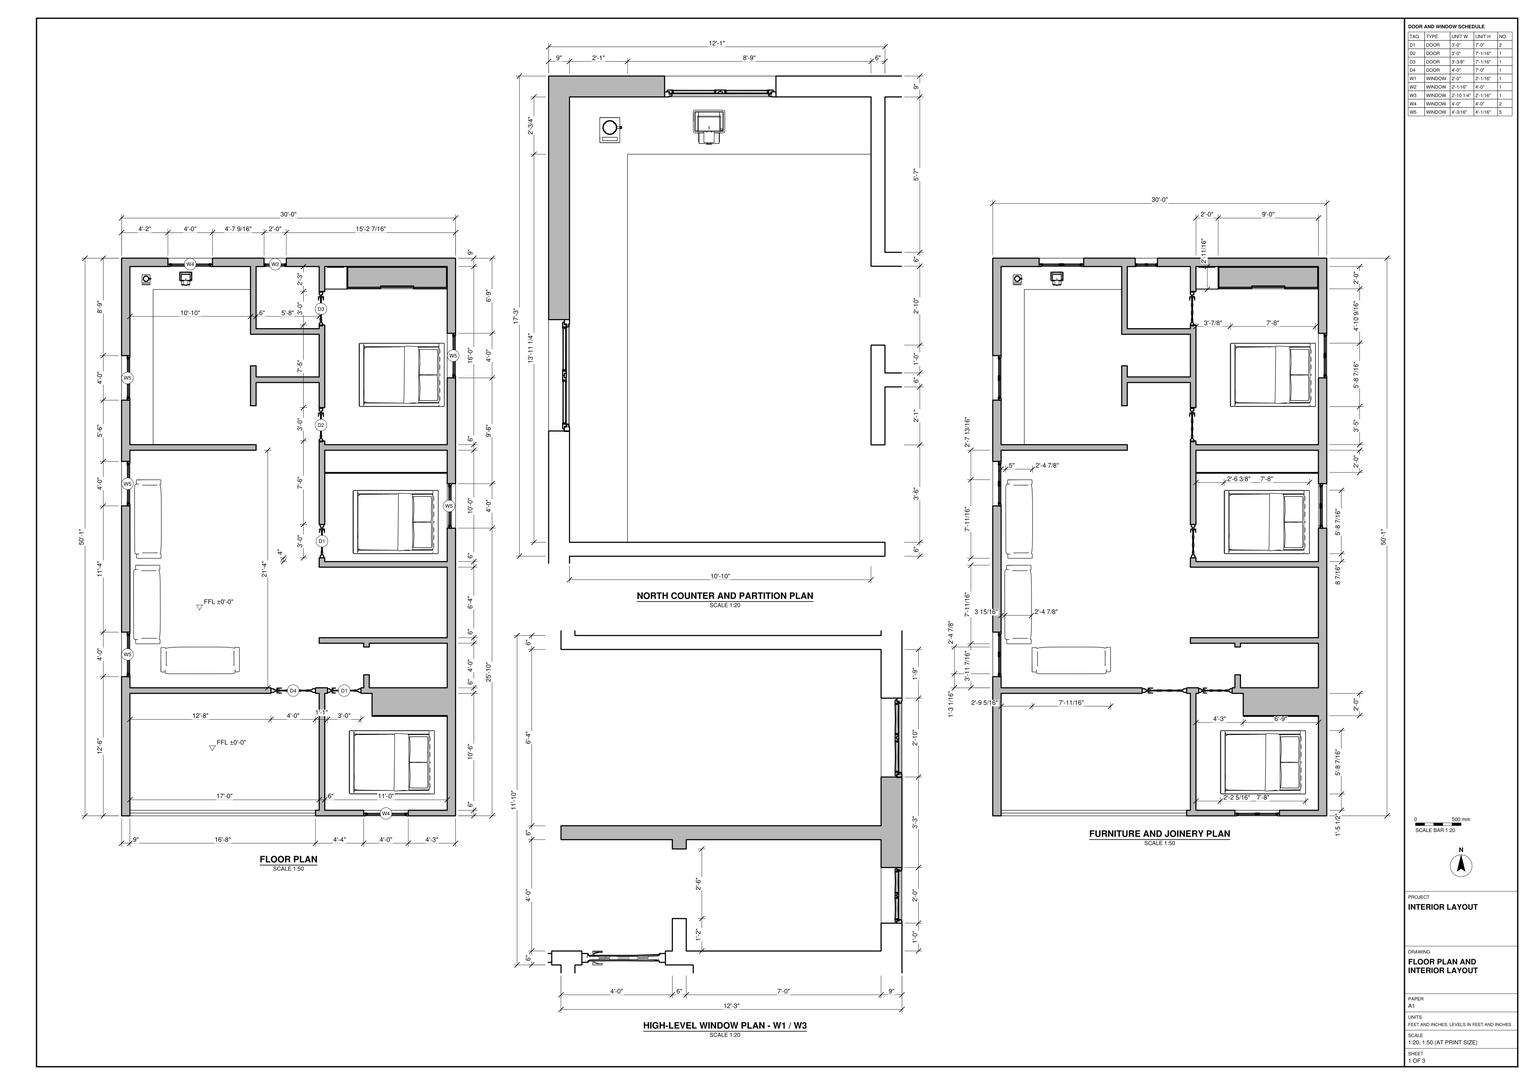
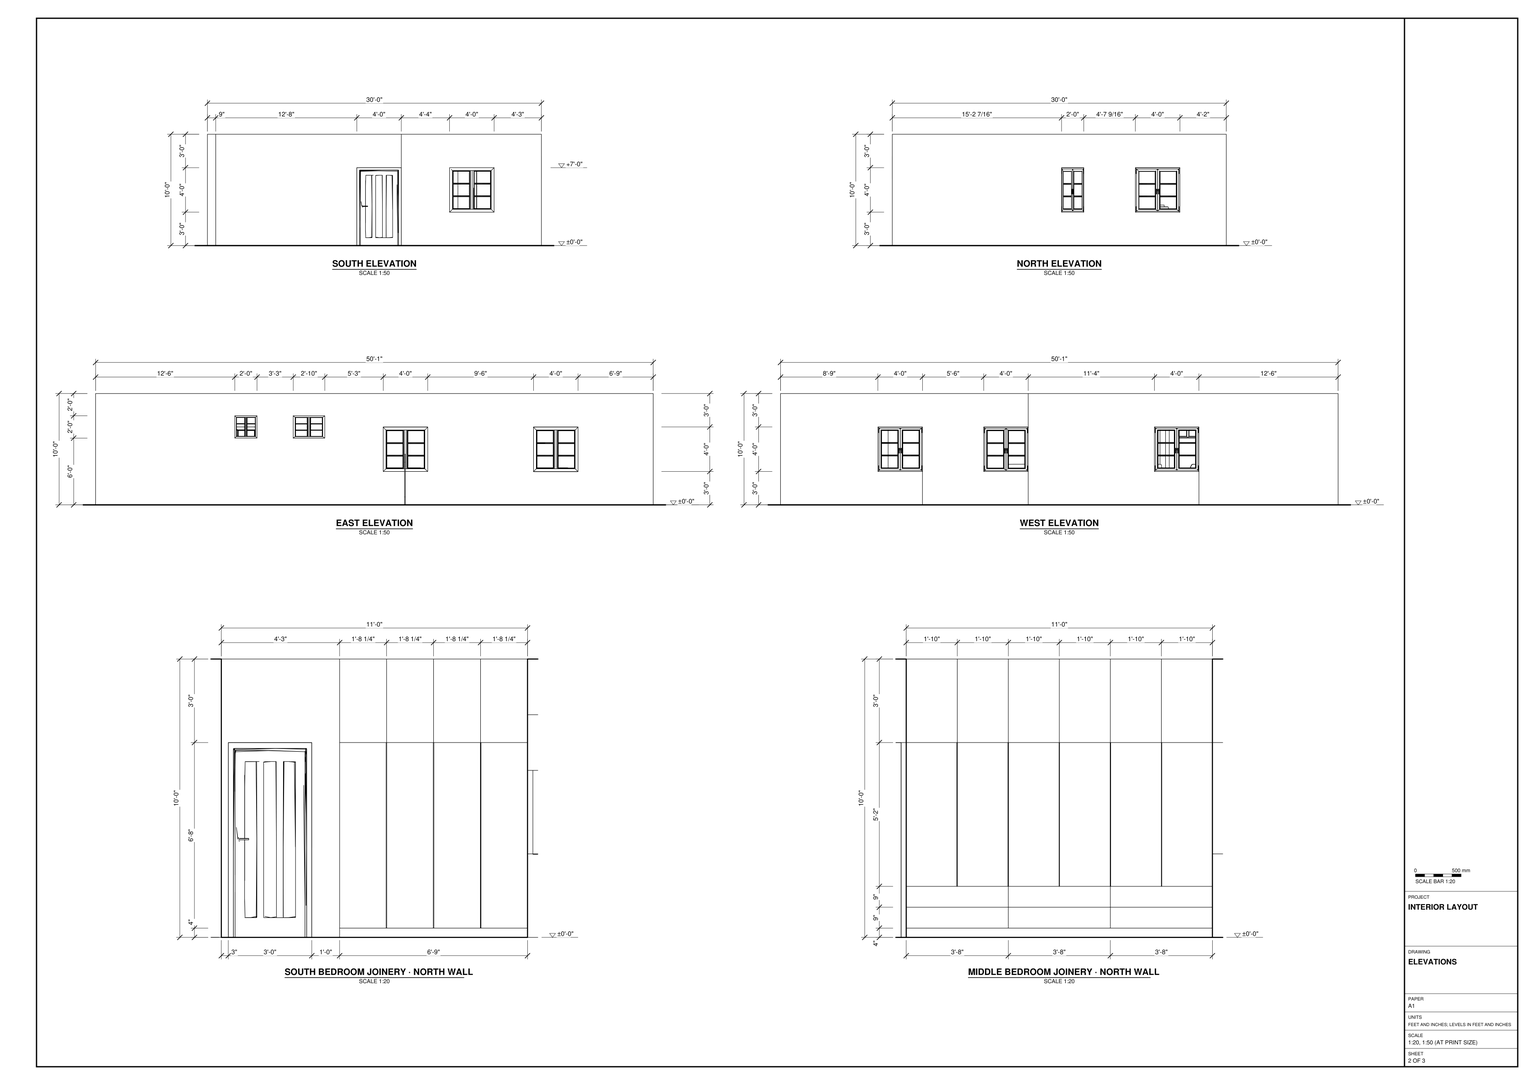
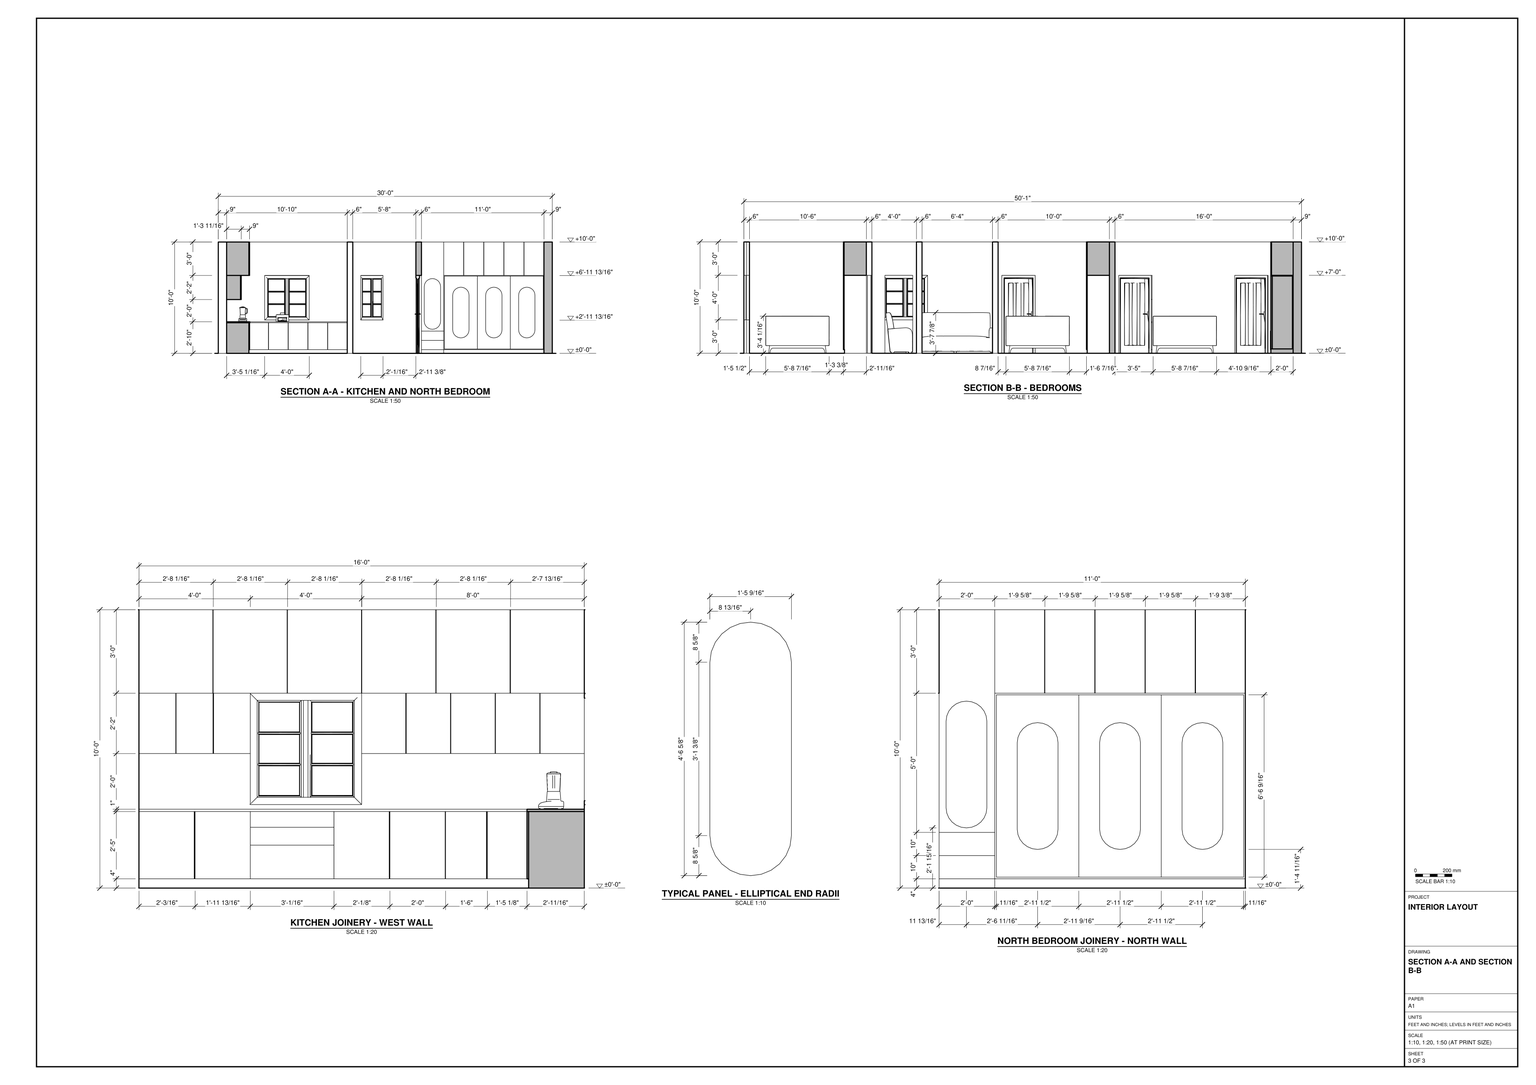
Build the single-storey interior in SketchUp from task_files/diagram_01.pdf. Work in feet and inches. The overall model extents are 163'-9 5/8" along x, 130'-11 3/8" along y and 10'-1/16" along z. Use the dimensioned floor plan, not those overall extents, to set out the 30'-0" by 50'-1" shell. Set the finished floor at ±0'-0".

Model the floor, perimeter walls and internal partitions, following the 9" and 6" wall thicknesses where indicated. Lay out the three bedrooms along the east side, the kitchen in the northwest corner, the living area to its south and the separate southwest bay. Fit the doors and window units into their openings. Use the elevations to distinguish the two high-level east windows from the larger bedroom windows.

Build the kitchen counter along the north and west walls and fit the base and overhead cabinets around the windows. Follow the separate joinery elevations for each bedroom: include the rounded-end panel details in the north bedroom, the low drawer rows in the middle bedroom and the storage fitted around the south bedroom doorway. Position the platform beds and sofas to match the furniture plan. Decor and loose items, including countertop appliances, may be any suitable library components.

Keep the shell elements and each furniture or joinery piece in separate groups or components, and use components for repeated parts. Save one SketchUp model as output_files/three_bedroom_interior_with_kitchen_and_bedroom_joinery.skp.

# SketchUp Ruby script. Lengths in inches.
U = 1.inch
M = Sketchup.active_model
def pt(a) = Geom::Point3d.new(a.map { |v| v * U })
def face(e, loops, mat)
  f = e.add_face(loops[0].map { |a| pt(a) })
  loops[1..].each { |l| e.add_face(l.map { |a| pt(a) }).erase! }
  f.material = f.back_material = mat if mat
  f
end
# faces: each face lists its corners as indices into pts; further lists are holes
def faces(e, pts, list, mat = nil) = list.each { |f| face(e, (f[0].is_a?(Array) ? f : [f]).map { |l| l.map { |i| pts[i] } }, mat) }
# xy, xz, yz: faces in a plane at the given z, y or x. An outline is a flat list of corners, or four numbers for a rectangle; further outlines are holes
def ring(l) = l.size == 4 ? [[l[0], l[1]], [l[2], l[1]], [l[2], l[3]], [l[0], l[3]]] : l.each_slice(2).to_a
def flat(e, list, mat, &to3) = list.each { |f| face(e, (f[0].is_a?(Array) ? f : [f]).map { |l| ring(l).map { |u, v| to3.(u, v) } }, mat) }
def xy(e, z, list, mat = nil) = flat(e, list, mat) { |x, y| [x, y, z] }
def xz(e, y, list, mat = nil) = flat(e, list, mat) { |x, z| [x, y, z] }
def yz(e, x, list, mat = nil) = flat(e, list, mat) { |y, z| [x, y, z] }
def lines(e, pts, list) = list.each { |a, b| e.add_line(pt(pts[a]), pt(pts[b])) }
# prism: a flat outline (further loops are holes) pulled along v
def prism(e, loops, v, mat = nil)
  f = face(e, loops, mat); d = Geom::Vector3d.new(v.map { |x| x * U })
  f.pushpull(f.normal.samedirection?(d) ? d.length : -d.length)
end
def box(e, o, s, mat = nil) = prism(e, [[o, [o[0] + s[0], o[1], o[2]], [o[0] + s[0], o[1] + s[1], o[2]], [o[0], o[1] + s[1], o[2]]]], [0, 0, s[2]], mat)
def at(x, y, z, deg = 0) = Geom::Transformation.translation(pt([x, y, z])) * Geom::Transformation.rotation(ORIGIN, Z_AXIS, deg.degrees)
def axes(o, x, y, z) = Geom::Transformation.new([*x, 0, *y, 0, *z, 0, *pt(o).to_a, 1])
def part(name) = M.definitions.add(name)
# library, detail: a bought-in or finely detailed component or shape, given as its bounding box
def library(name, o, s) = part(name).tap { |d| box(d.entities, o, s) }
def detail(e, o, s) = box(e.add_group.entities, o, s)
def put(e, d, t, mat = nil) = e.add_instance(d, t).tap { |i| i.material = mat if mat }
def group(e, t, mat = nil) = e.add_group.tap { |g| g.transformation = t; g.material = mat if mat }.entities
root = M.entities
M.materials.add("[Color C02]").color = [255, 204, 153]
M.materials.add("[Color M00]").color = [255, 255, 255]
M.materials.add("[Color M01]").color = [226, 226, 226]
M.materials.add("[Marble Carrara Floor Tile]").color = [204, 208, 219]
M.materials.add("[Marble Carrara Gold Floor Tile]").color = [225, 223, 217]
c1 = library("Tyler Platform Bed",[-34.22,-45.98,0],[68.44,91.98,40.05])
c2 = library("Sofa 142 022",[-42.35,-14.43,0],[84.7,28.86,43.89])
c3 = library("Blender 61-22",[-4.71,-5.45,0.07],[9.42,10.9,16.13])
c4 = library("Printer 12-16",[-6.8125,-7.36,0],[13.625,14.73,9.69])
c5 = library("Door 243 067",[-20.85,-3,0],[41.7,6,82.46])
c6 = library("Window 46-30",[-29.96,-2.6,0],[59.92,5.19,59.84])
c7 = part("Group\#6")
box(c7.entities,[0,0,0],[0.71,23.8,29])
c8 = part("Group\#1")
box(c8.entities,[0.2,0,0],[21,0.71,29])
c9 = part("Group\#17")
xy(c9.entities,0,[[0,0,35.53,1.5]])
xy(c9.entities,80,[[0,0,35.53,1.5]])
xz(c9.entities,0,[[17.76,12.1875,20.04,12.49,22.16,13.36,23.98,14.76,25.375,16.58,26.25,18.7,26.55,20.97,26.55,59.03,26.25,61.3,25.375,63.42,23.98,65.24,22.16,66.64,20.04,67.51,17.76,67.8125,15.49,67.51,13.37,66.64,11.55,65.24,10.15,63.42,9.27,61.3,8.97,59.03,8.97,20.97,9.27,18.7,10.15,16.58,11.55,14.76,13.37,13.36,15.49,12.49]],"[Color C02]")
xz(c9.entities,0,[[[0,0,35.53,80],[17.76,12.1875,15.49,12.49,13.37,13.36,11.55,14.76,10.15,16.58,9.27,18.7,8.97,20.97,8.97,59.03,9.27,61.3,10.15,63.42,11.55,65.24,13.37,66.64,15.49,67.51,17.76,67.8125,20.04,67.51,22.16,66.64,23.98,65.24,25.375,63.42,26.25,61.3,26.55,59.03,26.55,20.97,26.25,18.7,25.375,16.58,23.98,14.76,22.16,13.36,20.04,12.49]]],"[Color M01]")
xz(c9.entities,1.5,[[0,0,35.53,80]])
yz(c9.entities,0,[[0,0,1.5,80]])
yz(c9.entities,35.53,[[0,0,1.5,80]])
c10 = part("Group\#12")
box(c10.entities,[0.2,0,0],[21.4,0.71,36])
c11 = part("Group\#14")
box(c11.entities,[0,0,0],[24,0.71,10])
c12 = part("Group\#20")
box(c12.entities,[0.2,0,0],[20.05,0.71,80],"[Color M00]")
c13 = part("Group\#21")
box(c13.entities,[0,0,0],[20.25,0.71,36],"[Color M00]")
c14 = part("Group\#22")
box(c14.entities,[0,0,0],[44,0.71,9],"[Color M00]")
c15 = part("Group\#23")
box(c15.entities,[0,0,0],[21.8,0.71,62],"[Color M00]")
c16 = part("Group\#24")
box(c16.entities,[0,0,0],[22,0.71,36],"[Color M00]")
c17 = part("Group\#27")
box(c17.entities,[0,0.2,0],[0.71,31.8,36])
c18 = part("Group\#29")
box(c18.entities,[0,0.2,0],[0.71,15.8,26])
c19 = part("Group\#26")
box(c19.entities,[0,0,0],[0.71,19,26])
xy(root,0,[[[9.375,0,824.3125,0,814.9375,1571.375,0,1571.375],[95.5625,244.0625,455.5625,845.0625]],[[824.3125,0,1760.4375,0,1751.0625,1571.375,814.9375,1571.375],[1031.6875,244.0625,1391.6875,845.0625]],[95.5625,244.0625,104.5625,244.0625,104.5625,376.0625,256.5625,376.0625,256.5625,382.0625,104.5625,382.0625,104.5625,394.0625,95.5625,394.0625],[104.5625,244.0625,304.5625,247.0625],[304.5625,244.0625,356.5625,244.0625,356.5625,250.0625,314.5625,250.0625,314.5625,376.0625,317.5625,376.0625,317.5625,382.0625,304.5625,382.0625,304.5625,376.0625,308.5625,376.0625,308.5625,250.0625,304.5625,250.0625],
  [404.5625,244.0625,455.5625,244.0625,455.5625,394.0625,446.5625,394.0625,446.5625,382.0625,362.5625,382.0625,362.5625,396.0625,356.5625,396.0625,356.5625,382.0625,353.5625,382.0625,353.5625,376.0625,446.5625,376.0625,446.5625,250.0625,404.5625,250.0625],[356.5625,244.0625,404.5625,247.0625],[1040.6875,244.0625,1240.6875,247.0625],[104.5625,247.0625,304.5625,250.0625],[356.5625,247.0625,404.5625,250.0625],
  [1040.6875,247.0625,1240.6875,250.0625],[104.5625,250.0625,308.5625,250.0625,308.5625,376.0625,304.5625,376.0625,304.5625,382.0625,317.5625,382.0625,317.5625,376.0625,314.5625,376.0625,314.5625,250.0625,446.5625,250.0625,446.5625,376.0625,353.5625,376.0625,353.5625,382.0625,356.5625,382.0625,356.5625,396.0625,362.5625,396.0625,362.5625,382.0625,446.5625,382.0625,446.5625,430.0625,362.5625,430.0625,362.5625,426.0625,356.5625,426.0625,356.5625,430.0625,308.5625,430.0625,308.5625,436.0625,446.5625,436.0625,446.5625,512.0625,308.5625,512.0625,308.5625,522.0625,314.5625,522.0625,314.5625,518.0625,446.5625,518.0625,446.5625,638.0625,314.5625,638.0625,314.5625,558.0625,308.5625,558.0625,308.5625,648.0625,314.5625,648.0625,314.5625,644.0625,446.5625,644.0625,446.5625,836.0625,314.5625,836.0625,314.5625,809.0625,308.5625,809.0625,308.5625,836.0625,240.5625,836.0625,240.5625,769.0625,308.5625,769.0625,308.5625,773.0625,314.5625,773.0625,314.5625,684.0625,308.5625,684.0625,308.5625,711.0625,240.5625,711.0625,240.5625,686.0625,234.5625,686.0625,234.5625,729.0625,240.5625,729.0625,240.5625,717.0625,308.5625,717.0625,308.5625,763.0625,234.5625,763.0625,234.5625,812.0625,128.5625,812.0625,128.5625,644.0625,240.5625,644.0625,240.5625,638.0625,104.5625,638.0625,104.5625,382.0625,256.5625,382.0625,256.5625,376.0625,104.5625,376.0625],[95.5625,394.0625,100.0625,442.0625],[100.0625,394.0625,104.5625,442.0625],[446.5625,394.0625,451.0625,418.0625],
  [451.0625,394.0625,455.5625,418.0625],[446.5625,418.0625,455.5625,418.0625,455.5625,457.0625,446.5625,457.0625,446.5625,436.0625,308.5625,436.0625,308.5625,430.0625,356.5625,430.0625,356.5625,426.0625,362.5625,426.0625,362.5625,430.0625,446.5625,430.0625],[95.5625,442.0625,104.5625,578.0625],[446.5625,457.0625,451.0625,491.0625],[451.0625,457.0625,455.5625,491.0625],
  [446.5625,491.0625,455.5625,491.0625,455.5625,554.0625,446.5625,554.0625,446.5625,518.0625,314.5625,518.0625,314.5625,522.0625,308.5625,522.0625,308.5625,512.0625,446.5625,512.0625],[446.5625,554.0625,451.0625,602.0625],[451.0625,554.0625,455.5625,602.0625],[308.5625,558.0625,314.5625,558.0625,314.5625,638.0625,446.5625,638.0625,446.5625,602.0625,455.5625,602.0625,455.5625,716.0625,446.5625,716.0625,446.5625,644.0625,314.5625,644.0625,314.5625,648.0625,308.5625,648.0625],[1244.6875,558.0625,1250.6875,558.0625,1250.6875,638.0625,1382.6875,638.0625,1382.6875,602.0625,1391.6875,602.0625,1391.6875,764.0625,1382.6875,764.0625,1382.6875,644.0625,1250.6875,644.0625,1250.6875,648.0625,1244.6875,648.0625],
  [95.5625,578.0625,100.0625,626.0625],[100.0625,578.0625,104.5625,626.0625],[95.5625,626.0625,104.5625,626.0625,104.5625,638.0625,240.5625,638.0625,240.5625,644.0625,104.5625,644.0625,104.5625,692.0625,95.5625,692.0625],[104.5625,644.0625,128.5625,644.0625,128.5625,812.0625,234.5625,812.0625,234.5625,836.0625,104.5625,836.0625],[1040.6875,644.0625,1064.6875,644.0625,1064.6875,812.0625,1170.6875,812.0625,1170.6875,836.0625,1040.6875,836.0625],
  [308.5625,684.0625,314.5625,684.0625,314.5625,773.0625,308.5625,773.0625,308.5625,769.0625,240.5625,769.0625,240.5625,836.0625,249.125,836.0625,249.125,845.0625,193.5625,845.0625,193.5625,836.0625,234.5625,836.0625,234.5625,763.0625,308.5625,763.0625,308.5625,717.0625,240.5625,717.0625,240.5625,729.0625,234.5625,729.0625,234.5625,686.0625,240.5625,686.0625,240.5625,711.0625,308.5625,711.0625],[95.5625,692.0625,100.0625,740.0625],[100.0625,692.0625,104.5625,740.0625],[446.5625,716.0625,451.0625,764.0625],[451.0625,716.0625,455.5625,764.0625],
  [95.5625,740.0625,104.5625,740.0625,104.5625,836.0625,145.5625,836.0625,145.5625,845.0625,95.5625,845.0625],[446.5625,764.0625,455.5625,764.0625,455.5625,845.0625,273.125,845.0625,273.125,836.0625,308.5625,836.0625,308.5625,809.0625,314.5625,809.0625,314.5625,836.0625,446.5625,836.0625],[1382.6875,764.0625,1391.6875,764.0625,1391.6875,845.0625,1185.25,845.0625,1185.25,836.0625,1244.6875,836.0625,1244.6875,809.0625,1250.6875,809.0625,1250.6875,836.0625,1382.6875,836.0625],[1250.6875,812.0625,1274.6875,836.0625],[1274.6875,812.0625,1382.6875,836.0625],
  [145.5625,836.0625,193.5625,840.5625],[249.125,836.0625,273.125,840.5625],[145.5625,840.5625,193.5625,845.0625],[249.125,840.5625,273.125,845.0625]])
xy(root,0,[[1250.6875,614.0625,1382.6875,638.0625]],"[Color M00]")
xy(root,0,[[1040.6875,250.0625,1244.6875,250.0625,1244.6875,376.0625,1240.6875,376.0625,1240.6875,382.0625,1253.6875,382.0625,1253.6875,376.0625,1250.6875,376.0625,1250.6875,250.0625,1382.6875,250.0625,1382.6875,352.5,1301.6875,352.5,1301.6875,376.0625,1289.6875,376.0625,1289.6875,382.0625,1292.6875,382.0625,1292.6875,396.0625,1298.6875,396.0625,1298.6875,382.0625,1382.6875,382.0625,1382.6875,430.0625,1298.6875,430.0625,1298.6875,426.0625,1292.6875,426.0625,1292.6875,430.0625,1244.6875,430.0625,1244.6875,436.0625,1382.6875,436.0625,1382.6875,512.0625,1244.6875,512.0625,1244.6875,522.0625,1250.6875,522.0625,1250.6875,518.0625,1382.6875,518.0625,1382.6875,614.0625,1250.6875,614.0625,1250.6875,558.0625,1244.6875,558.0625,1244.6875,648.0625,1250.6875,648.0625,1250.6875,644.0625,1382.6875,644.0625,1382.6875,812.0625,1250.6875,812.0625,1250.6875,809.0625,1244.6875,809.0625,1244.6875,836.0625,1176.6875,836.0625,1176.6875,769.0625,1244.6875,769.0625,1244.6875,773.0625,1250.6875,773.0625,1250.6875,684.0625,1244.6875,684.0625,1244.6875,711.0625,1176.6875,711.0625,1176.6875,686.0625,1170.6875,686.0625,1170.6875,729.0625,1176.6875,729.0625,1176.6875,717.0625,1244.6875,717.0625,1244.6875,763.0625,1170.6875,763.0625,1170.6875,812.0625,1064.6875,812.0625,1064.6875,644.0625,1176.6875,644.0625,1176.6875,638.0625,1040.6875,638.0625,1040.6875,382.0625,1192.6875,382.0625,1192.6875,376.0625,1040.6875,376.0625]],"[Marble Carrara Gold Floor Tile]")
xy(root,4,[[1301.6875,352.0625,1382.6875,352.5]],"[Color M00]")
xy(root,36,[[1292.6875,244.0625,1340.6875,250.0625],[1031.6875,394.0625,1040.6875,442.0625],[1382.6875,554.0625,1391.6875,602.0625],[1031.6875,578.0625,1040.6875,626.0625],[1031.6875,692.0625,1040.6875,740.0625],
  [1382.6875,716.0625,1391.6875,764.0625],[1081.6875,836.0625,1129.6875,845.0625],[1185.25,836.0625,1209.25,845.0625]])
xy(root,58,[[1040.6875,644.0625,1052.6875,692.0625],[1040.6875,740.0625,1055.6875,836.0625]])
xy(root,72,[[1382.6875,394.0625,1391.6875,418.0625],[1382.6875,457.0625,1391.6875,491.0625]])
xy(root,84,[[1292.6875,244.0625,1340.6875,250.0625],[1192.6875,376.0625,1240.6875,376.9375],[1253.6875,376.0625,1289.6875,382.0625],[1192.6875,376.9375,1240.6875,382.0625],[1031.6875,394.0625,1040.6875,442.0625],
  [1292.6875,396.0625,1298.6875,426.0625],[1244.6875,522.0625,1250.6875,558.0625],[1382.6875,554.0625,1391.6875,602.0625],[1031.6875,578.0625,1040.6875,626.0625],[1170.6875,644.0625,1176.6875,686.0625],
  [1244.6875,648.0625,1250.6875,684.0625],[1031.6875,692.0625,1040.6875,740.0625],[1382.6875,716.0625,1391.6875,764.0625],[1170.6875,729.0625,1176.6875,763.0625],[1040.6875,740.0625,1055.6875,836.0625],
  [1244.6875,773.0625,1250.6875,809.0625],[1081.6875,836.0625,1129.6875,845.0625],[1185.25,836.0625,1209.25,845.0625]])
xy(root,84,[[1301.6875,352.0625,1382.6875,376.0625],[1250.6875,614.0625,1382.6875,638.0625]],"[Color M00]")
xy(root,84,[[1040.6875,644.0625,1052.6875,692.0625]],"[Color M01]")
xy(root,96,[[1382.6875,394.0625,1391.6875,418.0625],[1382.6875,457.0625,1391.6875,491.0625]])
xy(root,120,[[[1031.6875,244.0625,1040.6875,244.0625,1040.6875,376.0625,1244.6875,376.0625,1244.6875,250.0625,1240.6875,250.0625,1240.6875,244.0625,1391.6875,244.0625,1391.6875,845.0625,1031.6875,845.0625,1031.6875,578.0625,1040.6875,578.0625,1040.6875,638.0625,1176.6875,638.0625,1176.6875,711.0625,1244.6875,711.0625,1244.6875,512.0625,1382.6875,512.0625,1382.6875,436.0625,1244.6875,436.0625,1244.6875,430.0625,1292.6875,430.0625,1292.6875,382.0625,1040.6875,382.0625,1040.6875,578.0625,1031.6875,578.0625],[1250.6875,644.0625,1382.6875,836.0625],[1040.6875,644.0625,1170.6875,836.0625],[1250.6875,250.0625,1382.6875,376.0625],[1250.6875,518.0625,1382.6875,638.0625],[1176.6875,769.0625,1244.6875,836.0625],[1298.6875,382.0625,1382.6875,430.0625],[1176.6875,717.0625,1244.6875,763.0625]]])
xy(root,120,[[1301.6875,352.0625,1382.6875,376.0625],[1250.6875,614.0625,1382.6875,638.0625]],"[Color M00]")
xz(root,244.0625,[[1031.6875,0,1040.6875,120],[[1240.6875,0,1391.6875,120],[1292.6875,36,1340.6875,84]]])
xz(root,250.0625,[[1240.6875,0,1244.6875,120],[[1250.6875,0,1382.6875,120],[1292.6875,36,1340.6875,84]]])
xz(root,352.0625,[[1301.6875,4,1362.4375,84],[1362.4375,4,1382.6875,84],[1301.6875,84,1362.4375,120],[1362.4375,84,1382.6875,120]],"[Color M00]")
xz(root,352.5,[[1301.6875,0,1382.6875,4]],"[Color M00]")
xz(root,376.0625,[[1040.6875,0,1192.6875,0,1192.6875,84,1240.6875,84,1240.6875,0,1244.6875,0,1244.6875,120,1040.6875,120],[1250.6875,0,1253.6875,0,1253.6875,84,1289.6875,84,1289.6875,0,1301.6875,0,1301.6875,120,1250.6875,120]])
xz(root,376.0625,[[1301.6875,84,1382.6875,120]],"[Color M00]")
xz(root,382.0625,[[1040.6875,0,1040.6875,120,1292.6875,120,1292.6875,0,1289.6875,0,1289.6875,84,1253.6875,84,1253.6875,0,1240.6875,0,1240.6875,84,1192.6875,84,1192.6875,0],[1298.6875,0,1382.6875,120]])
xz(root,394.0625,[[1031.6875,0,1036.1875,36],[1031.6875,36,1036.1875,84],[1036.1875,36,1040.6875,84],[1382.6875,72,1391.6875,96]])
xz(root,396.0625,[[1292.6875,0,1298.6875,84]])
xz(root,418.0625,[[1382.6875,72,1387.1875,96],[1387.1875,72,1391.6875,96]])
xz(root,426.0625,[[1292.6875,0,1298.6875,84]])
xz(root,430.0625,[[1244.6875,0,1292.6875,120],[1298.6875,0,1382.6875,120]])
xz(root,436.0625,[[1244.6875,0,1382.6875,120]])
xz(root,442.0625,[[1031.6875,36,1040.6875,84]])
xz(root,457.0625,[[1382.6875,72,1391.6875,96]])
xz(root,491.0625,[[1382.6875,72,1387.1875,96],[1387.1875,72,1391.6875,96]])
xz(root,512.0625,[[1244.6875,0,1382.6875,120]])
xz(root,518.0625,[[1250.6875,0,1382.6875,120]])
xz(root,522.0625,[[1244.6875,0,1250.6875,84]])
xz(root,554.0625,[[1382.6875,36,1391.6875,84]])
xz(root,558.0625,[[1244.6875,0,1250.6875,84]])
xz(root,578.0625,[[1031.6875,0,1036.1875,36],[1036.1875,0,1040.6875,36],[1031.6875,36,1036.1875,84],[1036.1875,36,1040.6875,84],[1031.6875,84,1036.1875,120],
  [1036.1875,84,1040.6875,120]])
xz(root,602.0625,[[1382.6875,36,1387.1875,84],[1387.1875,36,1391.6875,84]])
xz(root,614.0625,[[1250.6875,0,1382.6875,4],[1250.6875,4,1294.6875,13],[1294.6875,4,1338.6875,13],[1338.6875,4,1382.6875,13],[1250.6875,13,1382.6875,22],
  [1250.6875,22,1272.6875,84],[1272.6875,22,1294.6875,84],[1294.6875,22,1338.6875,84],[1338.6875,22,1382.6875,84],[1250.6875,84,1272.6875,120],
  [1272.6875,84,1294.6875,120],[1294.6875,84,1338.6875,120],[1338.6875,84,1382.6875,120]],"[Color M00]")
xz(root,626.0625,[[1031.6875,36,1040.6875,84]])
xz(root,638.0625,[[1040.6875,0,1176.6875,120],[1250.6875,84,1382.6875,120]])
xz(root,638.0625,[[1250.6875,0,1382.6875,84]],"[Color M00]")
xz(root,644.0625,[[1040.6875,0,1040.6875,58,1052.6875,58,1052.6875,84,1040.6875,84,1040.6875,120,1064.6875,120,1064.6875,0],[1064.6875,0,1064.6875,120,1170.6875,120,1170.6875,84,1176.6875,84,1176.6875,0],[1250.6875,0,1382.6875,120],[1040.6875,58,1052.6875,84]])
xz(root,648.0625,[[1244.6875,0,1250.6875,84]])
xz(root,684.0625,[[1244.6875,0,1250.6875,84]])
xz(root,686.0625,[[1170.6875,0,1176.6875,84]])
xz(root,692.0625,[[1031.6875,0,1036.1875,36],[1031.6875,36,1036.1875,84],[1036.1875,36,1040.6875,84]])
xz(root,692.0625,[[1040.6875,58,1052.6875,84]],"[Color M01]")
xz(root,711.0625,[[1176.6875,0,1244.6875,120]])
xz(root,716.0625,[[1382.6875,36,1391.6875,84]])
xz(root,717.0625,[[1176.6875,0,1244.6875,120]])
xz(root,729.0625,[[1170.6875,0,1176.6875,84]])
xz(root,740.0625,[[1031.6875,36,1040.6875,84],[1040.6875,58,1055.6875,84]])
xz(root,763.0625,[[1170.6875,0,1244.6875,0,1244.6875,120,1176.6875,120,1176.6875,84,1170.6875,84]])
xz(root,764.0625,[[1382.6875,36,1387.1875,84],[1387.1875,36,1391.6875,84]])
xz(root,769.0625,[[1176.6875,0,1244.6875,120]])
xz(root,773.0625,[[1244.6875,0,1250.6875,84]])
xz(root,809.0625,[[1244.6875,0,1250.6875,84]])
xz(root,836.0625,[[[1040.6875,0,1170.6875,0,1170.6875,120,1040.6875,120,1040.6875,84,1055.6875,84,1055.6875,58,1040.6875,58],[1081.6875,36,1129.6875,84]],[[1176.6875,0,1244.6875,120],[1185.25,36,1209.25,84]],[1250.6875,0,1382.6875,120],[1040.6875,58,1055.6875,82],[1040.6875,82,1055.6875,84]])
xz(root,845.0625,[[[1031.6875,0,1391.6875,120],[1081.6875,36,1129.6875,84],[1185.25,36,1209.25,84]]])
yz(root,1031.6875,[[244.0625,0,244.0625,120,578.0625,120,578.0625,0,394.0625,0,394.0625,36,442.0625,36,442.0625,84,394.0625,84,394.0625,0],[578.0625,0,578.0625,36,626.0625,36,626.0625,84,578.0625,84,578.0625,120,845.0625,120,845.0625,0,692.0625,0,692.0625,36,740.0625,36,740.0625,84,692.0625,84,692.0625,0]])
yz(root,1040.6875,[[244.0625,0,247.0625,120],[247.0625,0,250.0625,120],[250.0625,0,376.0625,120],[[382.0625,0,578.0625,120],[394.0625,36,442.0625,84]],[578.0625,0,638.0625,0,638.0625,120,578.0625,120,578.0625,84,626.0625,84,626.0625,36,578.0625,36],
  [644.0625,0,836.0625,0,836.0625,58,740.0625,58,740.0625,36,692.0625,36,692.0625,58,644.0625,58],[644.0625,58,692.0625,84],[740.0625,58,836.0625,84],[644.0625,84,836.0625,120]])
yz(root,1052.6875,[[644.0625,58,676.0625,84],[676.0625,58,692.0625,84]])
yz(root,1055.6875,[[740.0625,58,759.26,84],[759.26,58,836.0625,84]])
yz(root,1081.6875,[[836.0625,36,840.5625,84],[840.5625,36,845.0625,84]])
yz(root,1129.6875,[[836.0625,36,845.0625,84]])
yz(root,1170.6875,[[686.0625,0,686.0625,84,644.0625,84,644.0625,120,763.0625,120,763.0625,84,729.0625,84,729.0625,0],[763.0625,0,812.0625,120],[812.0625,0,836.0625,120]])
yz(root,1176.6875,[[638.0625,0,644.0625,0,644.0625,84,686.0625,84,686.0625,0,711.0625,0,711.0625,120,638.0625,120],[717.0625,0,729.0625,0,729.0625,84,763.0625,84,763.0625,120,717.0625,120],[769.0625,0,836.0625,120]])
yz(root,1185.25,[[836.0625,36,840.5625,84],[840.5625,36,845.0625,84]])
yz(root,1192.6875,[[376.0625,0,382.0625,84]])
yz(root,1209.25,[[836.0625,36,845.0625,84]])
yz(root,1240.6875,[[244.0625,0,247.0625,120],[247.0625,0,250.0625,120],[376.0625,0,382.0625,84]])
yz(root,1244.6875,[[250.0625,0,376.0625,120],[430.0625,0,436.0625,120],[512.0625,0,512.0625,120,711.0625,120,711.0625,0,684.0625,0,684.0625,84,648.0625,84,648.0625,0,558.0625,0,558.0625,84,522.0625,84,522.0625,0],[717.0625,0,763.0625,120],[769.0625,0,769.0625,120,836.0625,120,836.0625,0,809.0625,0,809.0625,84,773.0625,84,773.0625,0]])
yz(root,1250.6875,[[250.0625,0,376.0625,120],[518.0625,0,522.0625,0,522.0625,84,558.0625,84,558.0625,0,614.0625,0,614.0625,120,518.0625,120],[644.0625,0,648.0625,0,648.0625,84,684.0625,84,684.0625,0,773.0625,0,773.0625,84,809.0625,84,809.0625,0,836.0625,0,836.0625,120,644.0625,120]])
yz(root,1250.6875,[[614.0625,0,638.0625,84],[614.0625,84,638.0625,120]],"[Color M00]")
yz(root,1253.6875,[[376.0625,0,382.0625,84]])
yz(root,1289.6875,[[376.0625,0,382.0625,84]])
yz(root,1292.6875,[[382.0625,0,382.0625,120,430.0625,120,430.0625,0,426.0625,0,426.0625,84,396.0625,84,396.0625,0],[244.0625,36,250.0625,84]])
yz(root,1298.6875,[[382.0625,0,396.0625,0,396.0625,84,426.0625,84,426.0625,0,430.0625,0,430.0625,120,382.0625,120]])
yz(root,1301.6875,[[352.5,0,352.5,4,352.0625,4,352.0625,84,376.0625,84,376.0625,0],[352.0625,84,376.0625,120]],"[Color M00]")
yz(root,1340.6875,[[244.0625,36,247.0625,84],[247.0625,36,250.0625,84]])
yz(root,1382.6875,[[250.0625,0,250.0625,120,352.0625,120,352.0625,4,352.5,4,352.5,0],[[382.0625,0,430.0625,120],[394.0625,72,418.0625,96]],[[436.0625,0,512.0625,120],[457.0625,72,491.0625,96]],[[518.0625,0,614.0625,120],[554.0625,36,602.0625,84]],[[644.0625,0,836.0625,120],[716.0625,36,764.0625,84]]])
yz(root,1382.6875,[[614.0625,0,638.0625,84],[352.0625,84,376.0625,120],[614.0625,84,638.0625,120]],"[Color M00]")
yz(root,1391.6875,[[[244.0625,0,845.0625,120],[716.0625,36,764.0625,84],[554.0625,36,602.0625,84],[457.0625,72,491.0625,96],[394.0625,72,418.0625,96]]])
p = [[1081.6875,836.0625,0],[1081.6875,840.5625,0],[1340.6875,247.0625,0],[1340.6875,247.0625,36],[1081.6875,840.5625,36],[1387.1875,764.0625,0],
  [1387.1875,764.0625,36],[1185.25,840.5625,0],[1185.25,840.5625,36],[1387.1875,602.0625,0],[1387.1875,602.0625,36],[1387.1875,491.0625,0],
  [1387.1875,491.0625,72],[1387.1875,418.0625,0],[1387.1875,418.0625,72],[1036.1875,394.0625,84],[1036.1875,394.0625,120],[1036.1875,394.0625,0],
  [1040.6875,394.0625,0],[1387.1875,418.0625,96],[1387.1875,418.0625,120],[1391.6875,418.0625,0],[1382.6875,418.0625,0],[1340.6875,247.0625,84],
  [1340.6875,247.0625,120],[1340.6875,244.0625,0],[1340.6875,250.0625,0],[1036.1875,692.0625,0],[1040.6875,692.0625,0],[1036.1875,692.0625,84],
  [1036.1875,692.0625,120],[1081.6875,845.0625,0],[1081.6875,840.5625,84],[1081.6875,840.5625,120],[1185.25,840.5625,84],[1185.25,840.5625,120],
  [1387.1875,764.0625,84],[1387.1875,764.0625,120],[1387.1875,602.0625,84],[1387.1875,602.0625,120],[1387.1875,491.0625,96],[1387.1875,491.0625,120],
  [1391.6875,491.0625,0],[1382.6875,491.0625,0]]
lines(root,p,[[0,1],[2,3],[1,4],[5,6],[7,8],[9,10],[11,12],[13,14],[15,16],[17,18],[19,20],[21,13],
  [13,22],[23,24],[25,2],[2,26],[27,28],[29,30],[31,1],[32,33],[34,35],[36,37],[38,39],[40,41],
  [42,11],[11,43]])
put(root,c1,at(1333.57,719.3125,0,-90))
put(root,c1,at(1322.95,301.79,0,-90))
put(root,c1,at(1327.03,560.72,0,-90))
put(root,c2,at(1059.03,471.82,0,90))
put(root,c2,at(1116.36,411.5625,0,-180))
put(root,c2,at(1060.13,563.93,0,90))
put(root,c3,at(1058.44,821.75,34))
put(root,c4,at(1100.85,823.02,34))
put(root,c5,axes([1216.6875,379.07,0],[1.15116,0,0],[0,1,0],[0,0,1.01862]))
put(root,c5,axes([1271.6875,379.07,0],[0.86337,0,0],[0,1,0],[0,0,1.01862]))
put(root,c5,axes([1247.69,540.0625,0],[0,-0.86337,0],[1,0,0],[0,0,1.01862]))
put(root,c5,axes([1246.58,665.17,-0.07],[0,-0.86337,0],[1,0,0],[0,0,1.01943]))
put(root,c5,axes([1246.58,790.35,-0.07],[0,-0.872,0],[1,0,0],[0,0,1.01943]))
put(root,c6,axes([1384.6,578,35.79],[0,-0.80441,0],[1,0,0],[0,0,0.80287]))
put(root,c6,axes([1389.1,740,35.79],[0,-0.80441,0],[1,0,0],[0,0,0.80287]))
put(root,c6,axes([1038.1,602,35.79],[0,-0.80441,0],[1,0,0],[0,0,0.80287]))
put(root,c6,axes([1038.1,417.96,36],[0,-0.80441,0],[1,0,0],[0,0,0.80287]))
put(root,c6,axes([1038.1,715.96,36],[0,-0.80441,0],[1,0,0],[0,0,0.80287]))
put(root,c6,axes([1389.11,473.99,71.95],[0,-0.57113,0],[1,0,0],[0,0,0.40187]))
put(root,c6,axes([1389.1,406.0625,72],[0,-0.40055,0],[1,0,0],[0,0,0.40187]))
put(root,c6,axes([1316.6875,246.65,36],[-0.8011,0,0],[0,-1,0],[0,0,0.80216]))
put(root,c6,axes([1105.72,838.65,35.79],[-0.8011,0,0],[0,-1,0],[0,0,0.80216]))
put(root,c6,axes([1197.27,838.65,35.79],[-0.40112,0,0],[0,-1,0],[0,0,0.80216]))
g1 = group(root,at(1040.6875,644.0625,0),"[Marble Carrara Floor Tile]")
xy(g1,0,[[0,0,0,192,130,192,130,168,24,168,24,0]])
xy(g1,33,[[0,0,24,0,24,168,130,168,130,192,0,192]])
xz(g1,0,[[0,0,24,33]])
xz(g1,168,[[24,4,87.6,33],[87.6,4,108.8,33],[108.8,4,130,33]])
xz(g1,168,[[24,0,130,4]],"[Color M01]")
xz(g1,192,[[0,0,41,33],[41,0,130,33]])
yz(g1,0,[[0,0,48,33],[48,0,192,33]])
yz(g1,24,[[0,4,24,33],[24,4,48,33],[48,4,84.09,33],[84.09,4,108,33],[108,4,132,33],
  [132,4,150,33],[150,4,168,33]])
yz(g1,24,[[0,0,168,4]],"[Color M01]")
yz(g1,130,[[168,0,192,33]])
put(g1,c7,at(24,84.0625,4),"[Color M01]")
g2 = group(g1,at(24,60.29,18.5),"[Color M01]")
box(g2,[0,-12.29,0],[0.71,36.09,7.71])
g3 = group(g1,at(24,125.49,4),"[Color M01]")
box(g3,[0,6.71,0],[0.71,17.59,29])
g4 = group(g1,at(24,60.29,26.21),"[Color M01]")
box(g4,[0,-12.29,0],[0.71,36.09,6.79])
g5 = group(g1,at(24,143.49,4),"[Color M01]")
box(g5,[0,6.71,0],[0.71,17.09,29])
put(g1,c8,at(108.8,167.29,4),"[Color M01]")
put(g1,c8,at(23.8,167.29,4),"[Color M01]")
put(g1,c8,at(66.3,167.29,4),"[Color M01]")
put(g1,c8,at(87.55,167.29,4),"[Color M01]")
put(g1,c7,at(24,0,4),"[Color M01]")
put(g1,c7,at(24,108.2,4),"[Color M01]")
g6 = group(g1,at(24,60.29,4),"[Color M01]")
box(g6,[0,-12.29,0],[0.71,36.09,14.5])
put(g1,c8,at(45.05,167.29,4),"[Color M01]")
put(g1,c7,at(24,24.2,4),"[Color M01]")
g7 = group(g1,at(0,0,33),"[Marble Carrara Gold Floor Tile]")
prism(g7,[[[25,0,0],[0,0,0],[0,48,0],[0,192,0],[41,192,0],[130,192,0],[130,167.29,0],[25,167.29,0]]],[0,0,1],"[Marble Carrara Floor Tile]")
g8 = group(root,at(1274.6875,812.0625,0),"[Color M01]")
xy(g8,0,[[0,0,108,24]])
xy(g8,4.71,[[0.71,0,107.29,1.5],[0.71,1.5,36.24,3],[36.24,1.5,71.76,3],[71.76,1.5,107.29,3],[0.71,3,107.29,23.25]])
xy(g8,83.29,[[0.71,0,107.29,23.25]])
xy(g8,84,[[0,0,108,24]])
xz(g8,0,[[0,0,108,4],[[0,4,108,84],[0.71,4.71,107.29,83.29]]])
xz(g8,23.25,[[0.71,4.71,107.29,83.29]])
xz(g8,24,[[0,0,108,84]])
yz(g8,0,[[0,0,24,84]])
yz(g8,0.71,[[0,4.71,23.25,83.29]])
yz(g8,107.29,[[0,4.71,23.25,83.29]])
yz(g8,108,[[0,0,24,84]])
g9 = group(g8,at(0.71,0.125,4.71))
xy(g9,0,[[0,0,35.53,1.5]])
xy(g9,78.58,[[0,0,35.53,1.5]])
xz(g9,0,[[17.76,11.97,20.04,12.26,22.16,13.125,23.98,14.5,25.375,16.29,26.25,18.37,26.55,20.6,26.55,57.98,26.25,60.21,25.375,62.3,23.98,64.08,22.16,65.46,20.04,66.32,17.76,66.61,15.49,66.32,13.37,65.46,11.55,64.08,10.15,62.3,9.27,60.21,8.97,57.98,8.97,20.6,9.27,18.37,10.15,16.29,11.55,14.5,13.37,13.125,15.49,12.26]],"[Color C02]")
xz(g9,0,[[[0,0,35.53,78.58],[17.76,11.97,15.49,12.26,13.37,13.125,11.55,14.5,10.15,16.29,9.27,18.37,8.97,20.6,8.97,57.98,9.27,60.21,10.15,62.3,11.55,64.08,13.37,65.46,15.49,66.32,17.76,66.61,20.04,66.32,22.16,65.46,23.98,64.08,25.375,62.3,26.25,60.21,26.55,57.98,26.55,20.6,26.25,18.37,25.375,16.29,23.98,14.5,22.16,13.125,20.04,12.26]]],"[Color M01]")
xz(g9,1.5,[[0,0,35.53,78.58]])
yz(g9,0,[[0,0,1.5,78.58]])
yz(g9,35.53,[[0,0,1.5,78.58]])
put(g8,c9,axes([71.76,0,4.71],[1,0,0],[0,1,0],[0,0,0.98228]))
put(g8,c9,axes([36.24,1.5,4.71],[1,0,0],[0,1,0],[0,0,0.98228]))
g10 = group(g8,at(0,0,84))
xy(g10,0,[[0,0.71,108,24]])
xy(g10,36,[[0,0.71,108,24]])
xz(g10,0.71,[[0,0,86.4,36],[86.4,0,108,36]])
xz(g10,24,[[0,0,108,36]])
yz(g10,0,[[0.71,0,24,36]])
yz(g10,108,[[0.71,0,24,36]])
put(g10,c10,at(64.75,0,0))
put(g10,c10,at(43.1,0,0))
put(g10,c10,at(86.4,0,0))
put(g10,c10,at(21.45,0,0))
put(g10,c10,at(-0.2,0,0))
g11 = group(root,at(1250.6875,811.35,0))
xy(g11,0,[[0,0.71,24,24.71]])
xy(g11,4.71,[[0.71,0.71,23.29,24]])
xy(g11,23.29,[[0.71,0.71,23.29,24]])
xy(g11,24,[[0,0.71,24,24.71]])
xz(g11,0.71,[[0,0,24,4],[[0,4,24,24],[0.71,4.71,23.29,23.29]]])
xz(g11,24,[[0.71,4.71,23.29,23.29]])
xz(g11,24.71,[[0,0,24,24]])
yz(g11,0,[[0.71,0,24.71,24]])
yz(g11,0.71,[[0.71,4.71,24,23.29]])
yz(g11,23.29,[[0.71,4.71,24,23.29]])
yz(g11,24,[[0.71,0,24.71,24]])
put(g11,c11,at(0,0,4))
put(g11,c11,at(0,0,14))
g12 = group(root,at(1948.06,577.85,0),"[Color M01]")
xz(g12,-0.71,[[8.79,0,11.0625,0.29,13.18,1.16,15,2.53,16.4,4.32,17.28,6.4,17.58,8.63,17.58,46.01,17.28,48.24,16.4,50.33,15,52.11,13.18,53.49,11.0625,54.35,8.79,54.64,6.51,54.35,4.39,53.49,2.57,52.11,1.18,50.33,0.3,48.24,0,46.01,0,8.63,0.3,6.4,1.18,4.32,2.57,2.53,4.39,1.16,6.51,0.29]],"[Color M01]")
xz(g12,0,[[8.79,0,6.51,0.29,4.39,1.16,2.57,2.53,1.18,4.32,0.3,6.4,0,8.63,0,46.01,0.3,48.24,1.18,50.33,2.57,52.11,4.39,53.49,6.51,54.35,8.79,54.64,11.0625,54.35,13.18,53.49,15,52.11,16.4,50.33,17.28,48.24,17.58,46.01,17.58,8.63,17.28,6.4,16.4,4.32,15,2.53,13.18,1.16,11.0625,0.29]],"[Color C02]")
yz(g12,0,[[-0.71,8.63,0,46.01]],"[Color C02]")
yz(g12,17.58,[[-0.71,8.63,0,46.01]],"[Color C02]")
p = [[6.51,0,0.29],[8.79,0,0],[8.79,-0.71,0],[6.51,-0.71,0.29],[11.0625,0,0.29],[11.0625,-0.71,0.29],
  [4.39,0,1.16],[4.39,-0.71,1.16],[13.18,0,1.16],[13.18,-0.71,1.16],[2.57,0,2.53],[2.57,-0.71,2.53],
  [15,0,2.53],[15,-0.71,2.53],[1.18,0,4.32],[1.18,-0.71,4.32],[16.4,0,4.32],[16.4,-0.71,4.32],
  [0.3,0,6.4],[0.3,-0.71,6.4],[17.28,0,6.4],[17.28,-0.71,6.4],[0,0,8.63],[0,-0.71,8.63],
  [17.58,0,8.63],[17.58,-0.71,8.63],[0.3,0,48.24],[0,0,46.01],[0,-0.71,46.01],[0.3,-0.71,48.24],
  [17.58,0,46.01],[17.28,0,48.24],[17.28,-0.71,48.24],[17.58,-0.71,46.01],[1.18,0,50.33],[1.18,-0.71,50.33],
  [16.4,0,50.33],[16.4,-0.71,50.33],[2.57,0,52.11],[2.57,-0.71,52.11],[15,0,52.11],[15,-0.71,52.11],
  [4.39,0,53.49],[4.39,-0.71,53.49],[13.18,0,53.49],[13.18,-0.71,53.49],[6.51,0,54.35],[6.51,-0.71,54.35],
  [11.0625,0,54.35],[11.0625,-0.71,54.35],[8.79,0,54.64],[8.79,-0.71,54.64]]
faces(g12,p,[[0,1,2,3],[1,4,5,2],[6,0,3,7],[4,8,9,5],[10,6,7,11],[8,12,13,9],[14,10,11,15],[12,16,17,13],
  [18,14,15,19],[16,20,21,17],[22,18,19,23],[20,24,25,21],[26,27,28,29],[30,31,32,33],[34,26,29,35],[31,36,37,32],
  [38,34,35,39],[36,40,41,37],[42,38,39,43],[40,44,45,41],[46,42,43,47],[44,48,49,45],[50,46,47,51],[48,50,51,49]],"[Color C02]")
g13 = group(root,at(1253.69,836.0625,25.95),"[Color M01]")
prism(g13,[[[0,0,8.63],[0,0,46.01],[0.3,0,48.24],[1.18,0,50.33],[2.57,0,52.11],[4.39,0,53.49],[6.51,0,54.35],[8.79,0,54.64],[11.0625,0,54.35],[13.18,0,53.49],[15,0,52.11],[16.4,0,50.33],[17.28,0,48.24],[17.58,0,46.01],[17.58,0,8.63],[17.28,0,6.4],[16.4,0,4.32],[15,0,2.53],[13.18,0,1.16],[11.0625,0,0.29],[8.79,0,0],[6.51,0,0.29],[4.39,0,1.16],[2.57,0,2.53],[1.18,0,4.32],[0.3,0,6.4]]],[0,-0.71,0],"[Color M01]")
put(root,c12,at(1362.4375,351.35,4))
put(root,c12,at(1342.12,351.35,4))
put(root,c12,at(1321.81,351.35,4))
put(root,c12,at(1301.49,351.35,4))
put(root,c13,at(1362.4375,351.35,84))
put(root,c13,at(1342.1875,351.35,84))
put(root,c13,at(1321.9375,351.35,84))
put(root,c13,at(1301.6875,351.35,84))
put(root,c14,at(1250.6875,613.35,4))
put(root,c14,at(1294.6875,613.35,4))
put(root,c14,at(1338.6875,613.35,4))
put(root,c14,at(1250.6875,613.35,13))
put(root,c14,at(1294.6875,613.35,13))
put(root,c14,at(1338.6875,613.35,13))
put(root,c15,at(1250.6875,613.35,22))
put(root,c15,at(1272.73,613.35,22))
put(root,c15,at(1294.77,613.35,22))
put(root,c15,at(1316.81,613.35,22))
put(root,c15,at(1338.84,613.35,22))
put(root,c15,at(1360.88,613.35,22))
put(root,c16,at(1250.6875,613.35,84))
put(root,c16,at(1272.6875,613.35,84))
put(root,c16,at(1294.6875,613.35,84))
put(root,c16,at(1316.6875,613.35,84))
put(root,c16,at(1338.6875,613.35,84))
put(root,c16,at(1360.6875,613.35,84))
g14 = group(root,at(1040.6875,644.0625,84),"[Color M01]")
xy(g14,0,[[0,0,24,48],[0,48,24,96],[0,96,24,192]])
xy(g14,36,[[0,0,24,192]])
xz(g14,0,[[0,0,24,36]])
xz(g14,192,[[0,0,24,36]])
yz(g14,0,[[0,0,192,36]])
yz(g14,24,[[0,0,160,36],[160,0,192,36]])
put(g14,c17,at(24,160,0))
put(g14,c17,at(24,127.96,0))
put(g14,c17,at(24,95.92,0))
put(g14,c17,at(24,63.88,0))
put(g14,c17,at(24,31.84,0))
put(g14,c17,at(24,-0.2,0))
put(root,c18,at(1052.6875,676.0625,58),"[Color M01]")
put(root,c18,at(1052.6875,659.96,58),"[Color M01]")
put(root,c18,at(1052.6875,643.87,58),"[Color M01]")
put(root,c19,at(1055.6875,740.0625,58))
put(root,c19,at(1055.6875,759.3125,58))
put(root,c19,at(1055.6875,778.5625,58))
put(root,c19,at(1055.6875,797.81,58))
put(root,c19,at(1055.6875,817.06,58))
